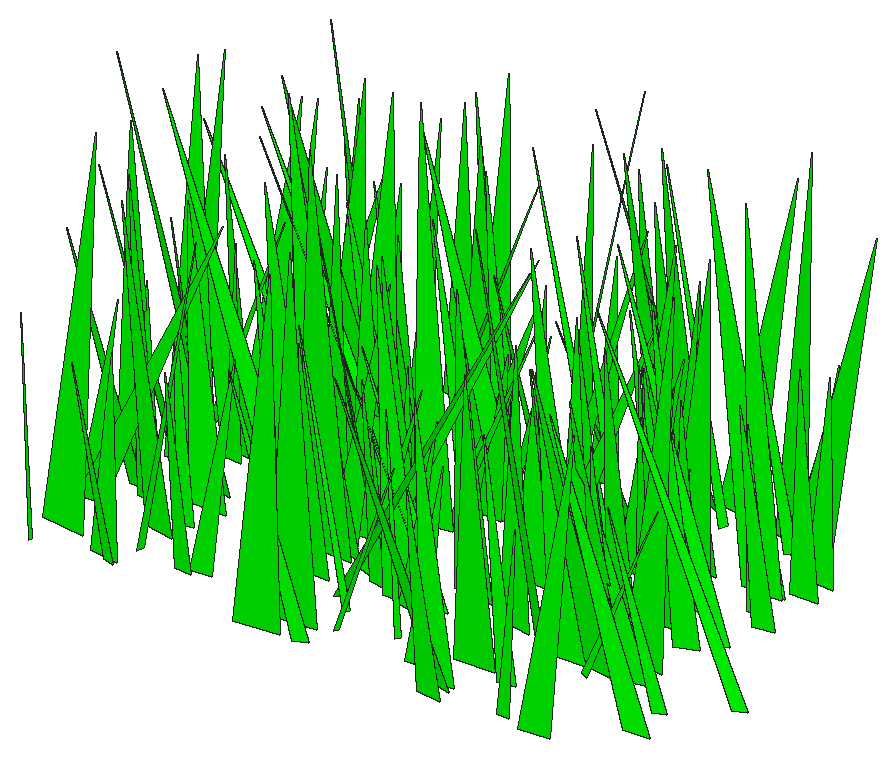
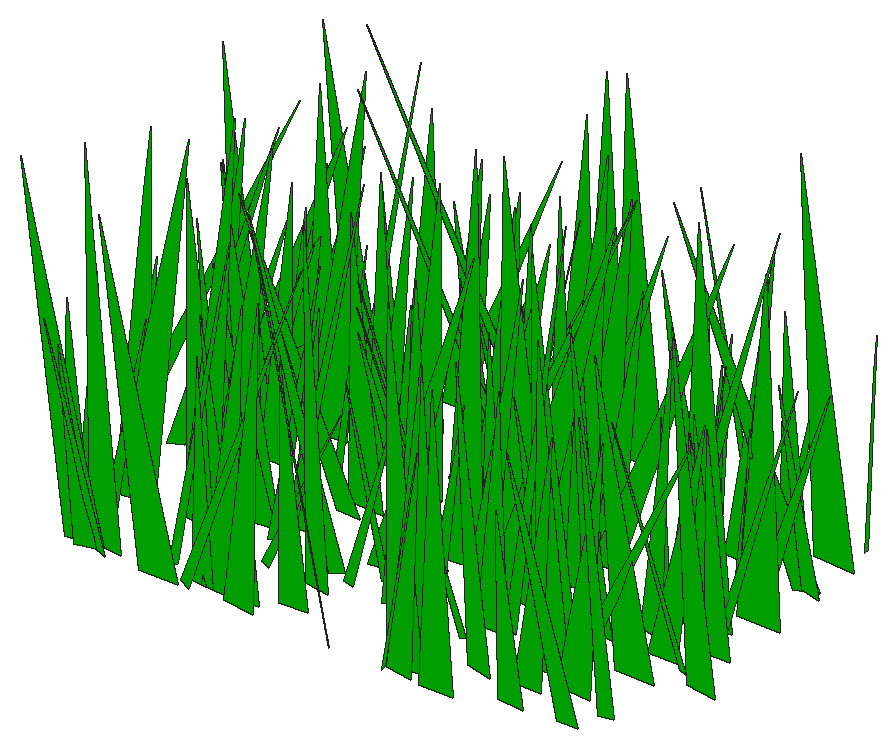
# SketchUp Ruby script. Lengths in inches.
U = 1.inch
M = Sketchup.active_model
def pt(a) = Geom::Point3d.new(a.map { |v| v * U })
def face(e, loops, mat)
  f = e.add_face(loops[0].map { |a| pt(a) })
  loops[1..].each { |l| e.add_face(l.map { |a| pt(a) }).erase! }
  f.material = f.back_material = mat if mat
  f
end
# faces: each face lists its corners as indices into pts; further lists are holes
def faces(e, pts, list, mat = nil) = list.each { |f| face(e, (f[0].is_a?(Array) ? f : [f]).map { |l| l.map { |i| pts[i] } }, mat) }
# xy, xz, yz: faces in a plane at the given z, y or x. An outline is a flat list of corners, or four numbers for a rectangle; further outlines are holes
def ring(l) = l.size == 4 ? [[l[0], l[1]], [l[2], l[1]], [l[2], l[3]], [l[0], l[3]]] : l.each_slice(2).to_a
def flat(e, list, mat, &to3) = list.each { |f| face(e, (f[0].is_a?(Array) ? f : [f]).map { |l| ring(l).map { |u, v| to3.(u, v) } }, mat) }
def xy(e, z, list, mat = nil) = flat(e, list, mat) { |x, y| [x, y, z] }
def xz(e, y, list, mat = nil) = flat(e, list, mat) { |x, z| [x, y, z] }
def yz(e, x, list, mat = nil) = flat(e, list, mat) { |y, z| [x, y, z] }
def lines(e, pts, list) = list.each { |a, b| e.add_line(pt(pts[a]), pt(pts[b])) }
# prism: a flat outline (further loops are holes) pulled along v
def prism(e, loops, v, mat = nil)
  f = face(e, loops, mat); d = Geom::Vector3d.new(v.map { |x| x * U })
  f.pushpull(f.normal.samedirection?(d) ? d.length : -d.length)
end
def box(e, o, s, mat = nil) = prism(e, [[o, [o[0] + s[0], o[1], o[2]], [o[0] + s[0], o[1] + s[1], o[2]], [o[0], o[1] + s[1], o[2]]]], [0, 0, s[2]], mat)
def at(x, y, z, deg = 0) = Geom::Transformation.translation(pt([x, y, z])) * Geom::Transformation.rotation(ORIGIN, Z_AXIS, deg.degrees)
def axes(o, x, y, z) = Geom::Transformation.new([*x, 0, *y, 0, *z, 0, *pt(o).to_a, 1])
def part(name) = M.definitions.add(name)
# library, detail: a bought-in or finely detailed component or shape, given as its bounding box
def library(name, o, s) = part(name).tap { |d| box(d.entities, o, s) }
def detail(e, o, s) = box(e.add_group.entities, o, s)
def put(e, d, t, mat = nil) = e.add_instance(d, t).tap { |i| i.material = mat if mat }
def group(e, t, mat = nil) = e.add_group.tap { |g| g.transformation = t; g.material = mat if mat }.entities
root = M.entities
M.materials.add("[0065_Lime]").color = [0, 255, 0]
c1 = part("fur_instance\#9")
p = [[0.8125,0,1.79],[0.67,-0.02,1.48],[0,-0.11,0],[0,0.11,0]]
faces(c1.entities,p,[[0,1,2,3]])
put(root,c1,axes([128.36,25.24,1.48],[-5.45124,-0.32206,0.7676],[2.29946,-0.7767,-0.11531],[0.9253,0.03278,4.80872]),"[0065_Lime]")
put(root,c1,axes([126.6,28.42,1.48],[5.12882,0.74401,1.9801],[-5.5488,0.76272,-0.09391],[-1.78081,-0.23378,5.99536]),"[0065_Lime]")
put(root,c1,axes([128.54,23.16,1.48],[-4.31629,-0.39679,0.67394],[2.89898,-0.60885,0.27259],[0.50606,0.10351,4.18665]),"[0065_Lime]")
put(root,c1,axes([127.85,24.11,1.48],[1.08619,-0.99599,1.9327],[7.45455,0.16965,0.15759],[-0.56153,0.32556,5.83067]),"[0065_Lime]")
put(root,c1,axes([127.54,26.47,1.48],[2.10825,-0.60106,0.67829],[4.31892,0.30556,0.19131],[-0.58236,0.09014,3.87429]),"[0065_Lime]")
put(root,c1,axes([128.09,18.58,1.48],[-4.44439,0.01057,1.45017],[-0.00633,-0.67246,0.15145],[1.7844,0.02395,3.61247]),"[0065_Lime]")
put(root,c1,axes([128.82,27.52,1.48],[-2.99851,0.64533,0.96949],[-4.73197,-0.42122,-0.28803],[0.34683,-0.16778,4.45205]),"[0065_Lime]")
put(root,c1,axes([127.74,21.73,1.48],[3.06893,0.44988,0.68966],[-3.20366,0.44443,-0.28225],[-0.83994,-0.05139,3.59636]),"[0065_Lime]")
put(root,c1,axes([128.4,23.83,1.48],[0.17576,0.57046,0.80638],[-4.17485,0.03016,-0.11276],[-0.18541,-0.13822,3.30336]),"[0065_Lime]")
put(root,c1,axes([127.85,31.45,1.48],[5.57575,-0.28147,1.60103],[2.05886,0.82786,0.13292],[-1.90989,0.0707,4.81735]),"[0065_Lime]")
put(root,c1,axes([130.6875,29.14,1.48],[-5.86785,0.27841,0.12264],[-1.98156,-0.8248,0.0118],[0.1475,-0.00485,5.03772]),"[0065_Lime]")
put(root,c1,axes([128.2,25.96,1.48],[2.54807,-0.57423,0.55117],[4.0935,0.36617,0.26221],[-0.63396,0.05641,3.90846]),"[0065_Lime]")
put(root,c1,axes([128.17,25.77,1.48],[2.92875,-0.42505,0.72874],[3.07965,0.42246,0.06769],[-0.6842,0.08211,3.42411]),"[0065_Lime]")
put(root,c1,axes([130.85,24.41,1.48],[-8.10297,-0.46867,1.41828],[3.46754,-1.15578,0.30983],[1.46302,0.14363,7.12083]),"[0065_Lime]")
put(root,c1,axes([129.54,30.89,1.48],[-1.42001,0.77168,1.18596],[-5.68122,-0.18941,-0.37084],[-0.09192,-0.21427,4.59902]),"[0065_Lime]")
put(root,c1,axes([128.37,19.81,1.48],[4.31222,0.99704,2.20864],[-7.47705,0.6347,0.05797],[-1.34606,-0.33151,6.75356]),"[0065_Lime]")
put(root,c1,axes([129.02,25.15,1.48],[-1.68815,1.16851,2.08849],[-8.66909,-0.25824,0.20513],[0.7688,-0.34605,6.89907]),"[0065_Lime]")
put(root,c1,axes([129.43,22.68,1.48],[-4.73045,-0.60516,2.06423],[4.70075,-0.70552,0.19659],[1.70015,0.26691,5.19988]),"[0065_Lime]")
put(root,c1,axes([127.78,27.81,1.48],[4.69949,0.22317,0.59515],[-1.63286,0.66556,0.16792],[-0.62575,-0.06067,4.03153]),"[0065_Lime]")
put(root,c1,axes([128.71,29,1.48],[1.61719,0.98586,0.66344],[-7.06138,0.22831,0.02011],[-0.15895,-0.11247,5.85645]),"[0065_Lime]")
put(root,c1,axes([130.15,24.52,1.48],[-5.25006,-0.05932,1.32609],[0.44112,-0.77227,-0.00207],[1.62525,0.01799,4.28425]),"[0065_Lime]")
put(root,c1,axes([130,26.58,1.48],[-4.6553,-0.52348,1.86225],[4.03781,-0.69497,0.1323],[1.67801,0.22004,4.84807]),"[0065_Lime]")
put(root,c1,axes([128.48,32.51,1.48],[4.50434,-0.44839,0.30422],[3.16327,0.63477,0.36214],[-0.56214,-0.02088,4.47549]),"[0065_Lime]")
put(root,c1,axes([129.81,26.1875,1.48],[3.15286,0.42847,1.30576],[-3.13439,0.48362,-0.3102],[-1.43187,-0.1152,3.55424]),"[0065_Lime]")
put(root,c1,axes([130.79,18.97,1.48],[-3.50978,-0.27197,0.77527],[1.97583,-0.50791,-0.05225],[0.86639,0.05654,3.25981]),"[0065_Lime]")
put(root,c1,axes([130.82,21.38,1.48],[4.14781,0.5827,3.14049],[-5.04503,0.68585,0.14447],[-2.57879,-0.40453,4.76863]),"[0065_Lime]")
put(root,c1,axes([131.07,23.4,1.48],[-2.52189,0.85597,0.41224],[-6.09526,-0.35795,0.23385],[0.46008,-0.05024,5.35769]),"[0065_Lime]")
put(root,c1,axes([130.82,31.52,1.48],[-2.64544,-0.67542,0.98386],[4.8913,-0.3869,-0.19837],[0.8014,0.13183,4.45844]),"[0065_Lime]")
put(root,c1,axes([127.97,21.64,1.48],[6.66383,-0.54985,0.25057],[3.92503,0.93408,-0.38047],[-0.02811,0.0786,6.27434]),"[0065_Lime]")
put(root,c1,axes([130.58,32.63,1.48],[1.2353,0.62221,0.22842],[-4.41369,0.17651,-0.31846],[-0.45299,-0.02306,3.72572]),"[0065_Lime]")
put(root,c1,axes([130.49,19.14,1.48],[-0.36437,-0.65465,0.72084],[4.71853,-0.06257,-0.32591],[0.47541,0.11922,3.78717]),"[0065_Lime]")
put(root,c1,axes([131.2,22.17,1.48],[-3.17769,0.35343,1.3892],[-2.7832,-0.47787,-0.13836],[1.22341,-0.16915,3.29356]),"[0065_Lime]")
put(root,c1,axes([133.64,24.24,1.48],[-7.57903,0.57656,0.67516],[-4.15104,-1.06628,-0.31904],[0.54158,-0.10416,7.00307]),"[0065_Lime]")
put(root,c1,axes([130.8,30.38,1.48],[-2.15852,-0.86634,2.15904],[6.58022,-0.35047,-0.35971],[1.3256,0.32905,5.30123]),"[0065_Lime]")
put(root,c1,axes([131.2,27.61,1.48],[3.68263,0.67698,1.88421],[-5.23663,0.5363,0.31501],[-1.0745,-0.29345,4.92251]),"[0065_Lime]")
put(root,c1,axes([131.0625,20.17,1.48],[6.95692,-0.07579,1.54226],[0.48327,1.01303,0.22578],[-1.91111,-0.01972,5.67134]),"[0065_Lime]")
put(root,c1,axes([131.97,28.79,1.48],[1.75237,1.02452,2.73925],[-8.02553,0.24154,0.36973],[-0.30105,-0.47562,6.08829]),"[0065_Lime]")
put(root,c1,axes([133.48,29,1.48],[-8.28885,-0.3976,2.24934],[2.96631,-1.22145,-0.0024],[2.61803,0.12512,7.12427]),"[0065_Lime]")
put(root,c1,axes([132.9,19.9375,1.48],[2.42802,0.38625,1.59046],[-3.03118,0.39836,-0.18002],[-1.48007,-0.18221,2.97779]),"[0065_Lime]")
put(root,c1,axes([132.6,31.63,1.48],[4.71926,0.595,1.6003],[-4.32945,0.70482,-0.33377],[-1.7482,-0.1393,5.14658]),"[0065_Lime]")
put(root,c1,axes([132.86,33.375,1.48],[2.03214,0.7695,2.25335],[-6.0814,0.30757,0.1091],[-0.82435,-0.37211,4.74997]),"[0065_Lime]")
put(root,c1,axes([134.77,27.49,1.48],[-3.75806,-1.17212,0.34915],[8.34936,-0.52538,0.3594],[-0.22718,0.08046,7.43314]),"[0065_Lime]")
put(root,c1,axes([132.4375,28.39,1.48],[2.6981,0.53249,1.11642],[-4.0007,0.38196,0.29243],[-0.48834,-0.18719,3.77258]),"[0065_Lime]")
put(root,c1,axes([133.34,25.8,1.48],[0.1532,0.77343,1.28708],[-5.72518,0.02636,-0.07996],[-0.14625,-0.22182,4.47814]),"[0065_Lime]")
put(root,c1,axes([134.52,22.97,1.48],[-3.94621,0.59331,1.08159],[-4.32623,-0.56993,0.03246],[0.93783,-0.13257,4.70084]),"[0065_Lime]")
put(root,c1,axes([133.875,29.41,1.48],[-0.08094,-0.73517,0.47348],[5.26331,-0.01276,-0.06879],[0.09409,0.08159,4.25563]),"[0065_Lime]")
put(root,c1,axes([134.42,33.22,1.48],[-4.5904,-0.63188,1.96974],[4.8409,-0.68414,0.11024],[1.62812,0.2526,5.22579]),"[0065_Lime]")
put(root,c1,axes([133.41,20.16,1.48],[3.63232,-0.46458,0.98328],[3.41846,0.52377,-0.06282],[-0.84031,0.12259,3.99473]),"[0065_Lime]")
put(root,c1,axes([135.1,24.17,1.48],[-3.49938,1.17401,1.64262],[-8.57881,-0.49611,-0.21066],[0.5351,-0.27603,7.365]),"[0065_Lime]")
put(root,c1,axes([134.98,33.26,1.48],[-4.75245,-0.01414,1.16828],[0.09917,-0.69763,-0.01596],[1.43636,0.00139,3.86654]),"[0065_Lime]")
put(root,c1,axes([135.32,22.67,1.48],[-2.95769,0.99939,1.26736],[-7.27233,-0.41694,-0.2121],[0.35229,-0.21639,6.26186]),"[0065_Lime]")
put(root,c1,axes([134.44,32.9,1.48],[-4.67427,0.69394,3.00823],[-5.62339,-0.74741,-0.00385],[2.53833,-0.37794,5.53104]),"[0065_Lime]")
put(root,c1,axes([135.6,30.11,1.48],[-4.36123,0.34477,0.96175],[-2.43956,-0.63396,0.29597],[1.21108,-0.03546,4.05959]),"[0065_Lime]")
put(root,c1,axes([138.16,24.81,1.48],[-8.89015,0.22048,0.36949],[-1.55097,-1.25017,0.30693],[0.51261,0.0412,7.33671]),"[0065_Lime]")
put(root,c1,axes([134.96,24.67,1.48],[-4.70284,-0.75655,2.49387],[5.78196,-0.73024,-0.20907],[2.22627,0.2984,5.8111]),"[0065_Lime]")
put(root,c1,axes([135.97,27.34,1.48],[4.00496,0.57308,3.15071],[-4.9743,0.67276,0.0831],[-2.62546,-0.40044,4.64874]),"[0065_Lime]")
put(root,c1,axes([135.25,26.1,1.48],[-0.69402,1.27225,1.6384],[-9.26074,-0.11098,0.29224],[0.52075,-0.27803,7.38048]),"[0065_Lime]")
put(root,c1,axes([135.48,23.5,1.48],[-0.33835,-1.31135,0.83045],[9.3855,-0.05051,-0.14273],[0.21339,0.14244,7.59462]),"[0065_Lime]")
put(root,c1,axes([136.32,23.8,1.48],[-3.83122,-0.46714,1.0048],[3.41134,-0.55528,-0.04437],[0.96975,0.1078,4.12578]),"[0065_Lime]")
put(root,c1,axes([138.82,24.18,1.48],[-8.63876,-0.18357,0.37521],[1.32637,-1.21408,0.30195],[0.4001,0.06133,7.10036]),"[0065_Lime]")
put(root,c1,axes([135.71,30.74,1.48],[-0.26996,-1.05243,0.85572],[7.55253,-0.04537,-0.29345],[0.40191,0.14572,6.0891]),"[0065_Lime]")
put(root,c1,axes([136.18,22.21,1.48],[-0.79092,-0.68718,0.91682],[5.01712,-0.11213,0.04733],[0.12103,0.15768,4.0293]),"[0065_Lime]")
put(root,c1,axes([136,24.99,1.48],[2.85773,-0.8638,1.57929],[6.33008,0.43248,0.34786],[-1.22023,0.22055,5.5032]),"[0065_Lime]")
put(root,c1,axes([137.65,24.6875,1.48],[-3.76968,0.88265,0.56209],[-6.31559,-0.53009,-0.1315],[0.21627,-0.09498,5.9574]),"[0065_Lime]")
put(root,c1,axes([134.28,30.31,1.48],[7.01785,-0.05302,0.68482],[0.32584,0.99158,0.36325],[-0.86315,-0.05677,5.7051]),"[0065_Lime]")
put(root,c1,axes([137.67,23.56,1.48],[-6.7579,-0.16863,1.42108],[1.30131,-0.97762,0.20707],[1.67303,0.07924,5.57912]),"[0065_Lime]")
put(root,c1,axes([135.72,24.1,1.48],[4.21917,-0.63978,1.0409],[4.66332,0.60292,-0.08883],[-0.78788,0.14252,5.04835]),"[0065_Lime]")
put(root,c1,axes([137.09,26.78,1.48],[6.02705,-0.77947,3.15316],[6.06159,0.94613,0.17133],[-3.00913,0.34467,6.66065]),"[0065_Lime]")
put(root,c1,axes([137.21,30.05,1.48],[-5.55638,0.37925,1.97179],[-2.9422,-0.8356,-0.10014],[2.12226,-0.16551,5.02361]),"[0065_Lime]")
put(root,c1,axes([138.84,28.45,1.48],[-6.37446,0.63056,0.9363],[-4.56279,-0.90215,-0.1946],[0.8016,-0.12085,6.338]),"[0065_Lime]")
put(root,c1,axes([138.37,18.75,1.48],[-4.79165,0.33154,0.73993],[-2.45477,-0.67561,-0.37398],[0.60704,-0.11505,4.32835]),"[0065_Lime]")
put(root,c1,axes([136.8,18.59,1.48],[2.78151,-1.08808,1.04594],[7.81848,0.40106,0.22365],[-0.69636,0.15673,6.68888]),"[0065_Lime]")
put(root,c1,axes([138.29,21.07,1.48],[-5.61406,0.06569,1.21809],[-0.454,-0.81646,0.09096],[1.50165,-0.00126,4.58145]),"[0065_Lime]")
put(root,c1,axes([137.44,19.53,1.48],[2.22292,-1.16486,0.92105],[8.33411,0.32281,0.3723],[-0.73878,0.13666,6.97133]),"[0065_Lime]")
put(root,c1,axes([138.01,22.92,1.48],[2.71872,0.37082,1.75239],[-3.04287,0.43848,0.01434],[-1.53174,-0.21289,3.08187]),"[0065_Lime]")
put(root,c1,axes([137.75,24.56,1.48],[-2.42503,0.42267,1.40972],[-3.27279,-0.37742,0.06691],[1.15769,-0.1816,3.14211]),"[0065_Lime]")
put(root,c1,axes([138.21,24.12,1.48],[-1.67977,-0.91727,1.23655],[6.69151,-0.2421,-0.00345],[0.38305,0.20672,5.48277]),"[0065_Lime]")
put(root,c1,axes([139.05,29.875,1.48],[-4.18446,-0.28435,0.70445],[2.05749,-0.59817,-0.00454],[0.78213,0.05226,3.78081]),"[0065_Lime]")
put(root,c1,axes([136.95,23.88,1.48],[3.86905,-0.32193,0.33896],[2.27198,0.54678,0.24263],[-0.51041,-0.00645,3.64943]),"[0065_Lime]")
put(root,c1,axes([136.73,28.93,1.48],[3.88915,-0.50848,0.16706],[3.62302,0.5466,-0.05695],[-0.10262,0.02687,4.32069]),"[0065_Lime]")
put(root,c1,axes([138.01,28.28,1.48],[0.68852,-0.57175,0.18428],[4.06611,0.09423,-0.25479],[0.27162,0.03865,3.34704]),"[0065_Lime]")
put(root,c1,axes([139.23,22.59,1.48],[-2.86725,0.88818,1.01026],[-6.418,-0.41025,0.03395],[0.55169,-0.15647,5.64557]),"[0065_Lime]")
put(root,c1,axes([137.15,33.2,1.48],[8.08828,0.15163,1.6887],[-1.17698,1.17098,0.20664],[-2.02217,-0.07507,6.63419]),"[0065_Lime]")
put(root,c1,axes([138.2,29.11,1.48],[3.64546,0.22719,0.75814],[-1.67978,0.52467,0.07574],[-0.81302,-0.06537,3.24293]),"[0065_Lime]")
put(root,c1,axes([137.33,27.34,1.48],[4.99002,0.22103,0.37885],[-1.58694,0.70349,0.07695],[-0.41558,-0.0324,4.25513]),"[0065_Lime]")
put(root,c1,axes([140.6,22.78,1.48],[-5.06703,0.2088,0.40276],[-1.48058,-0.71539,0.10324],[0.51087,-0.00238,4.29391]),"[0065_Lime]")
put(root,c1,axes([139.43,32.05,1.48],[1.53359,-0.665,1.11417],[4.91685,0.21934,-0.09095],[-0.31182,0.18808,4.04552]),"[0065_Lime]")
put(root,c1,axes([139.6,30.69,1.48],[-5.60504,-0.59916,2.78275],[4.68339,-0.88142,-0.11795],[2.81979,0.27297,5.72732]),"[0065_Lime]")
put(root,c1,axes([138.77,19.98,1.48],[4.08924,-0.06136,0.494],[0.4455,0.58077,-0.02277],[-0.60087,0.01301,3.34507]),"[0065_Lime]")
put(root,c1,axes([139.55,22.36,1.48],[3.03376,0.4013,0.85015],[-2.94135,0.4399,-0.0133],[-0.77256,-0.09894,3.38906]),"[0065_Lime]")
put(root,c1,axes([140.52,20.77,1.48],[-4.47223,0.05202,1.43831],[-0.37479,-0.67566,0.04788],[1.76728,-0.01164,3.6499]),"[0065_Lime]")
put(root,c1,axes([141.73,30.5,1.48],[-3.76423,-0.22333,0.22925],[1.60927,-0.52703,0.27901],[0.12499,0.05986,3.31187]),"[0065_Lime]")
put(root,c1,axes([137.21,23.31,1.48],[7.8875,0.53927,0.02505],[-3.83766,1.10834,-0.01505],[-0.03578,0.00044,7.1349]),"[0065_Lime]")
put(root,c1,axes([140.73,33.0625,1.48],[3.17582,0.69224,2.62582],[-5.60195,0.51416,-0.05916],[-1.81876,-0.3749,4.76728]),"[0065_Lime]")
put(root,c1,axes([140.7,24.2,1.48],[-1.44029,-0.92344,1.05727],[6.68188,-0.21138,-0.16404],[0.47877,0.17215,5.46992]),"[0065_Lime]")
put(root,c1,axes([142.86,32.97,1.48],[-7.63095,-0.29734,0.90151],[2.15036,-1.0821,0.08364],[1.04017,0.05567,6.4408]),"[0065_Lime]")
put(root,c1,axes([142.35,28.6,1.48],[-7.99783,0.16069,1.64925],[-1.20497,-1.15807,-0.08528],[1.99168,-0.05536,6.57115]),"[0065_Lime]")
put(root,c1,axes([140.71,32.7,1.48],[-0.05756,-0.59502,0.32102],[4.23889,-0.01251,-0.27442],[0.34414,0.05463,3.43376]),"[0065_Lime]")
put(root,c1,axes([137.5,21.6875,1.48],[9.32055,-0.09955,0.11406],[0.71362,1.3087,-0.30987],[-0.11083,0.05487,7.59701]),"[0065_Lime]")
put(root,c1,axes([141.79,32.7,1.48],[-1.88079,-0.81086,1.52437],[6.05183,-0.27033,0.12197],[0.43136,0.25713,4.93532]),"[0065_Lime]")
put(root,c1,axes([139.74,29.56,1.48],[6.76751,-0.28545,1.05814],[2.12138,0.96344,-0.26776],[-1.14836,0.09754,5.7412]),"[0065_Lime]")
put(root,c1,axes([143.42,19.18,1.48],[-5.3208,-0.49138,0.28207],[3.49964,-0.74897,-0.04242],[0.31846,0.02063,5.17888]),"[0065_Lime]")
put(root,c1,axes([142.5,29.09,1.48],[-6.01762,0.24074,1.3171],[-1.66505,-0.87564,0.32968],[1.66871,-0.00559,5.07863]),"[0065_Lime]")
put(root,c1,axes([141.54,25.92,1.48],[1.84042,0.84156,1.35913],[-6.18226,0.27378,-0.14163],[-0.66288,-0.21691,5.09437]),"[0065_Lime]")
put(root,c1,axes([142.19,28.16,1.48],[-1.68781,-0.61457,1.1254],[4.5606,-0.24711,0.00356],[0.49386,0.18161,3.81329]),"[0065_Lime]")
put(root,c1,axes([141.96,19.83,1.48],[2.98373,-0.47304,0.92503],[3.48243,0.43076,-0.05055],[-0.70627,0.12555,3.6587]),"[0065_Lime]")
put(root,c1,axes([142.45,32.66,1.48],[-2.50173,-0.51055,1.69137],[3.99343,-0.39317,-0.06866],[1.25588,0.23317,3.58756]),"[0065_Lime]")
put(root,c1,axes([143.18,19.33,1.48],[-1.85862,0.77123,0.86083],[-5.58582,-0.26205,-0.11249],[0.20619,-0.14715,4.71213]),"[0065_Lime]")
put(root,c1,axes([143.93,32.19,1.48],[-7.15098,0.0723,1.68896],[-0.61209,-1.04464,-0.21623],[2.04974,-0.05971,5.82773]),"[0065_Lime]")
put(root,c1,axes([142.82,23.49,1.48],[-2.57099,-0.7457,1.62449],[5.51851,-0.39986,-0.37193],[1.30258,0.22222,4.78209]),"[0065_Lime]")
put(root,c1,axes([143.46,24.87,1.48],[-4.6568,-0.25007,1.2225],[1.73994,-0.6873,-0.32586],[1.54873,0.02023,4.04197]),"[0065_Lime]")
put(root,c1,axes([143.13,30.31,1.48],[-2.83228,-0.38138,1.404],[3.00196,-0.42947,0.09767],[1.15488,0.18104,3.18933]),"[0065_Lime]")
put(root,c1,axes([143.47,18.54,1.48],[-1.59035,-0.5801,0.6608],[4.18969,-0.22955,-0.08087],[0.38628,0.10139,3.59765]),"[0065_Lime]")
put(root,c1,axes([144.15,29.61,1.48],[4.91892,0.72235,4.17053],[-6.53915,0.81892,0.35006],[-3.15496,-0.57113,5.77676]),"[0065_Lime]")
put(root,c1,axes([144.61,22.64,1.48],[-8.05399,-0.32415,1.97907],[2.51515,-1.17237,0.33786],[2.21702,0.15245,6.80627]),"[0065_Lime]")
put(root,c1,axes([143.38,20.87,1.48],[0.97986,-1.0015,0.02947],[7.12171,0.13778,0.22849],[-0.28322,-0.00034,5.84746]),"[0065_Lime]")
put(root,c1,axes([141.69,26.57,1.48],[4.76872,0.65009,0.29204],[-4.64033,0.66794,0.31015],[0.00863,-0.07358,5.39552]),"[0065_Lime]")
put(root,c1,axes([143.42,30.38,1.48],[2.97411,0.4889,1.26661],[-3.71198,0.43457,0.14617],[-0.86672,-0.18352,3.72027]),"[0065_Lime]")
put(root,c1,axes([144.9,29.75,1.48],[-5.48609,-0.93137,2.09107],[6.86658,-0.81238,-0.20532],[1.84138,0.25455,6.9956]),"[0065_Lime]")
put(root,c1,axes([145.24,23.21,1.48],[-4.90998,0.90104,1.90706],[-6.70854,-0.7121,-0.15375],[1.26871,-0.27831,6.5675]),"[0065_Lime]")
put(root,c1,axes([144.85,20.5625,1.48],[-4.15469,0.38142,1.27536],[-2.82004,-0.61452,0.08015],[1.36885,-0.10832,4.03602]),"[0065_Lime]")
put(root,c1,axes([143.69,28.26,1.48],[3.3567,0.88285,1.76162],[-6.60481,0.48091,0.2508],[-0.73535,-0.2895,5.78875]),"[0065_Lime]")
put(root,c1,axes([143.36,28.65,1.48],[3.00974,-0.61448,0.43724],[4.40314,0.42273,-0.14664],[-0.15532,0.07662,4.3156]),"[0065_Lime]")
put(root,c1,axes([143.76,33.14,1.48],[2.84408,0.99566,1.16502],[-7.2257,0.39806,0.27156],[-0.21778,-0.20438,6.20459]),"[0065_Lime]")
put(root,c1,axes([144.32,29.33,1.48],[4.7455,0.51623,1.80697],[-3.98306,0.70303,0.1908],[-1.60214,-0.21873,4.87786]),"[0065_Lime]")
put(root,c1,axes([145.46,27.55,1.48],[1.42104,-0.56506,1.88252],[4.4913,0.25287,0.30025],[-1.16419,0.28581,3.45619]),"[0065_Lime]")
put(root,c1,axes([145.4,25.44,1.48],[-2.03036,-0.79425,1.12817],[5.77489,-0.30059,-0.21464],[0.72329,0.17038,4.88059]),"[0065_Lime]")
put(root,c1,axes([145.43,26.58,1.48],[-3.48879,-0.49567,1.61002],[3.77144,-0.53138,-0.0746],[1.46183,0.18796,4.03491]),"[0065_Lime]")
put(root,c1,axes([146.02,26.57,1.48],[4.82664,-0.33869,2.81163],[3.02352,0.79277,-0.23411],[-2.93531,0.25966,4.38213]),"[0065_Lime]")
put(root,c1,axes([144.875,29.39,1.48],[1.6387,-0.93695,1.57685],[6.94165,0.22825,-0.22839],[-0.17895,0.27409,5.58045]),"[0065_Lime]")
put(root,c1,axes([146.61,22.89,1.48],[-3.78561,-0.75174,0.48067],[5.36072,-0.53569,-0.13915],[0.48144,0.05382,5.32904]),"[0065_Lime]")
put(root,c1,axes([145.57,22.9,1.48],[3.92255,-0.77295,2.54692],[6.09132,0.60164,-0.08876],[-1.71979,0.36799,5.49474]),"[0065_Lime]")
put(root,c1,axes([146.58,32.15,1.48],[-4.60148,0.25707,1.07503],[-1.91887,-0.66763,-0.08466],[1.18806,-0.08266,4.02698]),"[0065_Lime]")
put(root,c1,axes([146.34,26.35,1.48],[-1.09836,-0.65021,0.32349],[4.6408,-0.15588,-0.07357],[0.18014,0.05142,3.86774]),"[0065_Lime]")
put(root,c1,axes([146.65,23.41,1.48],[-0.83434,-0.86279,0.06962],[6.13639,-0.11669,0.19757],[-0.22918,0.0165,5.03644]),"[0065_Lime]")
put(root,c1,axes([147.38,29.8,1.48],[-5.27132,0.9578,1.18037],[-6.90034,-0.75314,0.08929],[0.97572,-0.15172,7.00838]),"[0065_Lime]")
put(root,c1,axes([146.01,18.98,1.48],[3.07214,0.34377,0.98804],[-2.44727,0.46051,-0.33444],[-1.21308,-0.05844,3.17692]),"[0065_Lime]")
put(root,c1,axes([146.22,27.62,1.48],[0.91335,-0.60791,0.99794],[4.47214,0.1412,0.1742],[-0.47058,0.16203,3.59237]),"[0065_Lime]")
put(root,c1,axes([146.46,23.28,1.48],[0.67856,-0.63558,1.09197],[4.69128,0.11119,0.23982],[-0.50262,0.17976,3.71259]),"[0065_Lime]")
put(root,c1,axes([148.48,26.39,1.48],[-7.65611,0.30342,1.00888],[-2.19249,-1.08851,-0.03867],[1.18065,-0.05381,6.47041]),"[0065_Lime]")
put(root,c1,axes([146.12,32.74,1.48],[5.69283,0.77985,2.66503],[-6.07139,0.855,0.19728],[-2.1618,-0.34762,6.46396]),"[0065_Lime]")
put(root,c1,axes([147.95,23.07,1.48],[-2.59388,0.49572,0.21607],[-3.53449,-0.36112,-0.31216],[-0.15301,-0.06196,3.54805]),"[0065_Lime]")
put(root,c1,axes([147.73,25.66,1.48],[5.24908,-0.5183,2.80752],[3.97392,0.85549,0.37626],[-3.11867,0.21773,5.20482]),"[0065_Lime]")
put(root,c1,axes([147.5,29.71,1.48],[-5.88351,0.71598,2.22502],[-5.35118,-0.88194,0.14759],[2.1931,-0.23114,6.32923]),"[0065_Lime]")
put(root,c1,axes([146.125,33.01,1.48],[4.23651,0.3252,0.58281],[-2.2721,0.60372,-0.36012],[-0.84072,0.00713,3.91013]),"[0065_Lime]")
put(root,c1,axes([146.67,33.02,1.48],[2.13102,-0.46333,1.09577],[3.5441,0.29784,-0.34024],[-0.35565,0.19181,3.17529]),"[0065_Lime]")
put(root,c1,axes([146.61,25.09,1.48],[5.41704,-0.23678,1.40494],[1.64282,0.79877,0.32007],[-1.76746,0.01673,4.60344]),"[0065_Lime]")
put(root,c1,axes([146.33,22.49,1.48],[4.10476,0.19482,0.29519],[-1.39176,0.57879,0.00438],[-0.34209,-0.01704,3.52419]),"[0065_Lime]")
put(root,c1,axes([148.11,28.64,1.48],[-1.7338,0.52812,0.15068],[-3.7439,-0.24498,0.26921],[0.37818,-0.00406,3.35596]),"[0065_Lime]")
put(root,c1,axes([147.34,24.05,1.48],[3.65296,0.95742,2.12275],[-7.2172,0.53435,0.14151],[-1.07096,-0.3353,6.28692]),"[0065_Lime]")
put(root,c1,axes([149.8125,20.65,1.48],[-5.09666,0.57127,0.0049],[-4.06009,-0.71529,0.26716],[0.20952,0.03555,5.29633]),"[0065_Lime]")
put(root,c1,axes([147.39,18.75,1.48],[-3.88014,0.60298,3.1476],[-5.105,-0.66456,0.1022],[2.70683,-0.38898,4.70471]),"[0065_Lime]")
put(root,c1,axes([146.83,32.84,1.48],[4.91423,-0.88243,0.51366],[6.28618,0.69438,0.18126],[-0.56506,0.0505,6.4837]),"[0065_Lime]")
put(root,c1,axes([148.79,28.04,1.48],[-2.71813,0.48533,1.2485],[-3.71093,-0.39309,-0.22516],[0.71694,-0.19463,3.56798]),"[0065_Lime]")
put(root,c1,axes([148.58,30.26,1.48],[-1.50588,0.61966,1.20338],[-4.62168,-0.22398,0.03808],[0.52455,-0.19449,3.79018]),"[0065_Lime]")
put(root,c1,axes([151.38,23.68,1.48],[-7.66585,0.2913,0.23149],[-2.07107,-1.07793,0.07524],[0.29887,0.00212,6.45905]),"[0065_Lime]")
put(root,c1,axes([148.4375,31.23,1.48],[-0.08935,0.61445,1.00882],[-4.54229,-0.01834,0.10815],[0.16349,-0.17376,3.55595]),"[0065_Lime]")
put(root,c1,axes([149.58,22.04,1.48],[-3.52033,0.29006,0.52702],[-2.11705,-0.49767,-0.17821],[0.44591,-0.07287,3.31466]),"[0065_Lime]")
